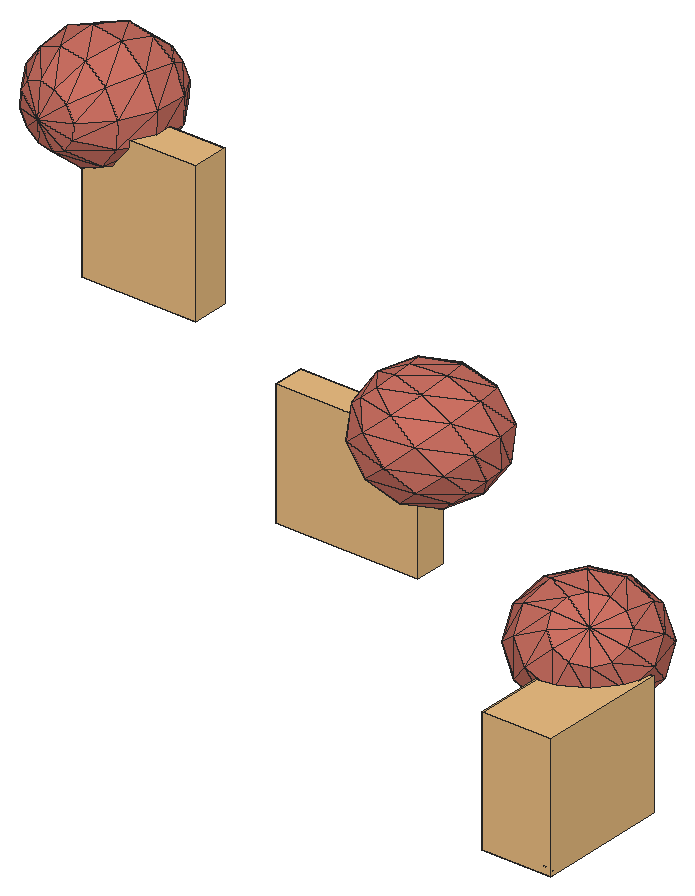
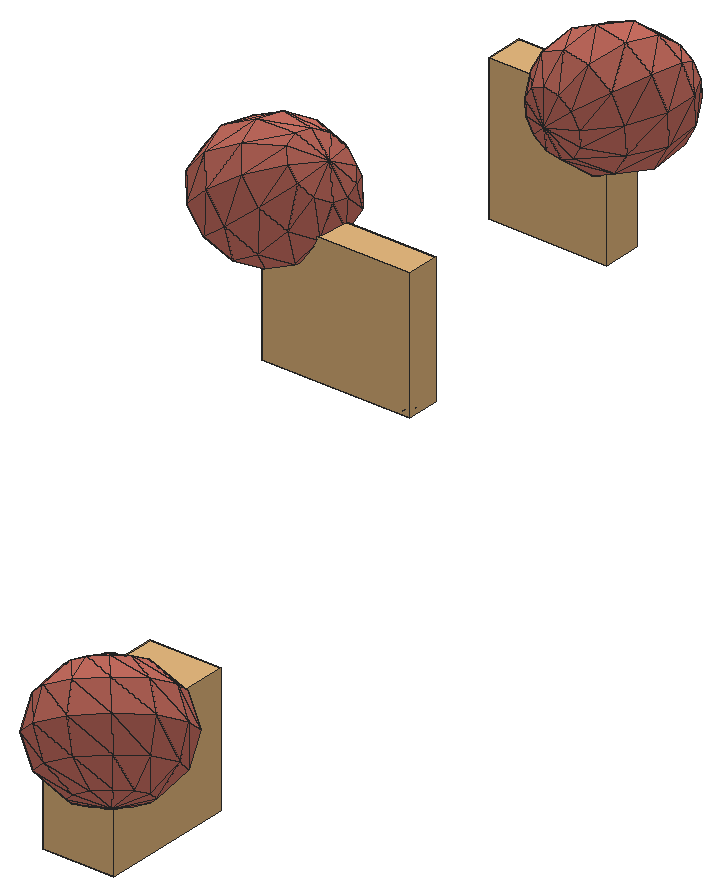
# SketchUp Ruby script. Lengths in inches.
U = 1.inch
M = Sketchup.active_model
def pt(a) = Geom::Point3d.new(a.map { |v| v * U })
def face(e, loops, mat)
  f = e.add_face(loops[0].map { |a| pt(a) })
  loops[1..].each { |l| e.add_face(l.map { |a| pt(a) }).erase! }
  f.material = f.back_material = mat if mat
  f
end
# faces: each face lists its corners as indices into pts; further lists are holes
def faces(e, pts, list, mat = nil) = list.each { |f| face(e, (f[0].is_a?(Array) ? f : [f]).map { |l| l.map { |i| pts[i] } }, mat) }
# xy, xz, yz: faces in a plane at the given z, y or x. An outline is a flat list of corners, or four numbers for a rectangle; further outlines are holes
def ring(l) = l.size == 4 ? [[l[0], l[1]], [l[2], l[1]], [l[2], l[3]], [l[0], l[3]]] : l.each_slice(2).to_a
def flat(e, list, mat, &to3) = list.each { |f| face(e, (f[0].is_a?(Array) ? f : [f]).map { |l| ring(l).map { |u, v| to3.(u, v) } }, mat) }
def xy(e, z, list, mat = nil) = flat(e, list, mat) { |x, y| [x, y, z] }
def xz(e, y, list, mat = nil) = flat(e, list, mat) { |x, z| [x, y, z] }
def yz(e, x, list, mat = nil) = flat(e, list, mat) { |y, z| [x, y, z] }
def lines(e, pts, list) = list.each { |a, b| e.add_line(pt(pts[a]), pt(pts[b])) }
# prism: a flat outline (further loops are holes) pulled along v
def prism(e, loops, v, mat = nil)
  f = face(e, loops, mat); d = Geom::Vector3d.new(v.map { |x| x * U })
  f.pushpull(f.normal.samedirection?(d) ? d.length : -d.length)
end
def box(e, o, s, mat = nil) = prism(e, [[o, [o[0] + s[0], o[1], o[2]], [o[0] + s[0], o[1] + s[1], o[2]], [o[0], o[1] + s[1], o[2]]]], [0, 0, s[2]], mat)
def at(x, y, z, deg = 0) = Geom::Transformation.translation(pt([x, y, z])) * Geom::Transformation.rotation(ORIGIN, Z_AXIS, deg.degrees)
def axes(o, x, y, z) = Geom::Transformation.new([*x, 0, *y, 0, *z, 0, *pt(o).to_a, 1])
def part(name) = M.definitions.add(name)
# library, detail: a bought-in or finely detailed component or shape, given as its bounding box
def library(name, o, s) = part(name).tap { |d| box(d.entities, o, s) }
def detail(e, o, s) = box(e.add_group.entities, o, s)
def put(e, d, t, mat = nil) = e.add_instance(d, t).tap { |i| i.material = mat if mat }
def group(e, t, mat = nil) = e.add_group.tap { |g| g.transformation = t; g.material = mat if mat }.entities
root = M.entities
M.materials.add("green").color = [174, 139, 102]
M.materials.add("vio").color = [206, 114, 100]
c1 = library("3DGeom~47_Defintion",[-132.29,-500,-408.57],[264.58,1000,817.14])
c2 = part("3DGeom~48_Defintion")
p = [[-103.8,487.39,-408.57],[-132.29,492.93,-365.46],[-123.73,496.1875,-348.87],[-103.8,487.39,-408.57],[-131.22,489.88,-384.15],[-132.29,492.93,-365.46],
  [-103.8,487.39,-408.57],[-120.79,487.85,-399.93],[-131.22,489.88,-384.15],[-103.8,487.39,-408.57],[-123.73,496.1875,-348.87],[-107.82,498.77,-338.8125],
  [-103.8,487.39,-408.57],[-107.82,498.77,-338.8125],[-88.83,500,-338],[-103.8,487.39,-408.57],[-60.34,494.46,-381.11],[-68.9,491.2,-397.7],
  [-103.8,487.39,-408.57],[-68.9,491.2,-397.7],[-84.8125,488.61,-407.76],[-103.8,487.39,-408.57],[-71.84,499.54,-346.64],[-61.42,497.51,-362.41],
  [-103.8,487.39,-408.57],[-61.42,497.51,-362.41],[-60.34,494.46,-381.11],[-103.8,487.39,-408.57],[-88.83,500,-338],[-71.84,499.54,-346.64],
  [91.01,-500,353.89],[109.71,-496.86,353.62],[124.82,-489.05,360.72],[62.5,-490.37,374.27],[91.01,-500,353.89],[67.8125,-469.79,401.48],
  [91.01,-500,353.89],[62.5,-490.37,374.27],[73.73,-497.625,361.44],[91.01,-500,353.89],[101.625,-458.84,408.31],[130.13,-468.47,387.93],
  [91.01,-500,353.89],[124.82,-489.05,360.72],[91.01,-500,353.89],[130.13,-468.47,387.93],[130.13,-468.47,387.93],[124.82,-489.05,360.72],
  [132.29,-478.66,373.28],[62.5,-490.37,374.27],[60.34,-480.18,388.92],[130.13,-468.47,387.93],[118.9,-461.21,400.75],[82.93,-461.98,408.57]]
faces(c2.entities,p,[[0,1,2],[3,4,5],[6,7,8],[9,10,11],[12,13,14],[15,16,17],[18,19,20],[21,22,23],
  [24,25,26],[27,28,29],[30,31,32],[33,34,35],[36,37,38],[35,39,40],[41,42,43],[40,44,45],
  [46,47,48],[49,35,50],[40,51,52],[35,40,53]],"green")
c3 = part("3DGeom~199_Defintion")
p = [[-69.55,-302.43,-360.84],[-338.74,-97.12,-366.25],[-102.46,-106.03,-485.67],[189.77,-256.61,-366.85],[161.26,-86.52,-474.95],[-343.46,97.57,-361.65],
  [-107.92,118.79,-480.36],[156.54,108.18,-470.35],[-323.15,264.7,-245.58],[-84.47,311.77,-346.33],[-323.15,264.7,-245.58],[-84.47,311.77,-346.33],
  [398.24,-142.03,-274.56],[398.24,-142.03,-274.56],[381.78,-43.83,-336.97],[381.78,-43.83,-336.97],[381.78,-43.83,-336.97],[379.05,68.57,-334.3125],
  [379.05,68.57,-334.3125],[176.85,275.3,-354.28],[-84.47,311.77,-346.33],[176.85,275.3,-354.28],[234.41,-356.52,-175.01],[-69.55,-302.43,-360.84],
  [189.77,-256.61,-366.85],[424.01,-199.72,-163.8],[234.41,-356.52,-175.01],[189.77,-256.61,-366.85],[189.77,-256.61,-366.85],[398.24,-142.03,-274.56],
  [-310.23,-267.21,-258.15],[-310.23,-267.21,-258.15],[-484.24,-62.19,-148.7],[-338.74,-97.12,-366.25],[-338.74,-97.12,-366.25],[-486.97,50.21,-146.04],
  [-338.74,-97.12,-366.25],[-343.46,97.57,-361.65],[-343.46,97.57,-361.65],[-475.25,146.71,-79.03],[-343.46,97.57,-361.65],[-323.15,264.7,-245.58],
  [-18,-417.8,-139.33],[-310.23,-267.21,-258.15],[-69.55,-302.43,-360.84],[234.41,-356.52,-175.01],[-69.55,-302.43,-360.84],[379.05,68.57,-334.3125],
  [176.85,275.3,-354.28],[390.78,165.07,-267.3],[390.78,165.07,-267.3],[176.85,275.3,-354.28],[216.77,370.09,-157.85],[176.85,275.3,-354.28],
  [-84.47,311.77,-346.33],[-38.375,421.22,-119.51],[176.85,275.3,-354.28],[216.77,370.09,-157.85],[-323.15,264.7,-245.58],[-283.23,359.48,-49.15],
  [381.78,-43.83,-336.97],[500,10.6,-108.7],[379.05,68.57,-334.3125],[413.82,219.79,-153.89],[-265.59,-367.12,-66.32],[-310.23,-267.21,-258.15],
  [-265.59,-367.12,-66.32],[-467.79,-160.39,-86.29],[-310.23,-267.21,-258.15],[-310.23,-267.21,-258.15],[-323.15,264.7,-245.58],[-452.2,201.43,34.38],
  [-323.15,264.7,-245.58],[-283.23,359.48,-49.15],[283.23,-359.48,49.15],[234.41,-356.52,-175.01],[452.2,-201.43,-34.38],[283.23,-359.48,49.15],
  [265.59,367.12,66.32],[216.77,370.09,-157.85],[18,417.8,139.33],[265.59,367.12,66.32],[216.77,370.09,-157.85],[442.01,218.08,-24.47],
  [-500,-10.6,108.7],[38.375,-421.22,119.51],[283.23,-359.48,49.15],[-234.41,356.52,175.02],[475.25,-146.71,79.03],[486.97,-50.21,146.04],
  [484.24,62.19,148.7],[467.79,160.39,86.29],[-265.59,-367.12,-66.32],[-442.01,-218.08,24.47],[-216.77,-370.09,157.85],[-216.77,-370.09,157.85],
  [-265.59,-367.12,-66.32],[-283.23,359.48,-49.15],[-424.01,199.72,163.8],[-283.23,359.48,-49.15],[-234.41,356.52,175.02],[310.23,267.21,258.15],
  [-216.77,-370.09,157.85],[-413.82,-219.79,153.89],[323.15,-264.7,245.59],[283.23,-359.48,49.15],[323.15,-264.7,245.59],[265.59,367.12,66.32],
  [69.55,302.43,360.84],[310.23,267.21,258.15],[265.59,367.12,66.32],[69.55,302.43,360.84],[338.74,97.12,366.25],[-390.78,-165.07,267.3],
  [-390.78,-165.07,267.3],[-379.05,-68.57,334.3125],[-379.05,-68.57,334.3125],[-381.78,43.83,336.97],[-381.78,43.83,336.97],[-398.24,142.03,274.56],
  [-398.24,142.03,274.56],[84.47,-311.77,346.34],[323.15,-264.7,245.59],[84.47,-311.77,346.34],[-189.77,256.61,366.85],[-189.77,256.61,366.85],
  [69.55,302.43,360.84],[343.46,-97.57,361.65],[-176.85,-275.3,354.28],[-216.77,-370.09,157.85],[-176.85,-275.3,354.28],[-390.78,-165.07,267.3],
  [84.47,-311.77,346.34],[-176.85,-275.3,354.28],[-234.41,356.52,175.02],[-398.24,142.03,274.56],[-234.41,356.52,175.02],[-398.24,142.03,274.56],
  [-189.77,256.61,366.85],[343.46,-97.57,361.65],[84.47,-311.77,346.34],[323.15,-264.7,245.59],[310.23,267.21,258.15],[102.46,106.03,485.67],
  [338.74,97.12,366.25],[310.23,267.21,258.15],[69.55,302.43,360.84],[-156.54,-108.17,470.35],[-390.78,-165.07,267.3],[-176.85,-275.3,354.28],
  [-379.05,-68.57,334.3125],[-189.77,256.61,366.85],[-398.24,142.03,274.56],[-381.78,43.83,336.97],[-161.26,86.52,474.95],[107.92,-118.79,480.36],
  [343.46,-97.57,361.65],[338.74,97.12,366.25],[343.46,-97.57,361.65],[338.74,97.12,366.25]]
faces(c3.entities,p,[[0,1,2],[3,0,2],[3,2,4],[2,1,5],[2,5,6],[4,2,6],[4,6,7],[6,5,8],
  [7,6,9],[6,10,11],[12,3,4],[13,4,14],[15,4,7],[16,7,17],[18,7,19],[7,20,21],
  [22,23,24],[25,26,27],[25,28,29],[0,30,1],[31,32,33],[34,32,35],[36,35,37],[38,35,39],
  [40,39,41],[42,43,44],[45,42,46],[47,48,49],[50,51,52],[53,54,55],[56,55,57],[54,58,59],
  [54,59,55],[29,60,61],[60,62,61],[62,50,61],[25,29,61],[50,63,61],[50,52,63],[42,64,65],
  [66,67,68],[69,67,32],[70,39,71],[72,71,73],[74,42,75],[76,77,26],[76,26,25],[76,25,61],
  [63,52,78],[79,80,81],[82,55,80],[63,83,61],[63,78,83],[32,67,84],[35,32,84],[39,35,84],
  [85,64,42],[86,85,42],[55,59,87],[55,87,80],[88,76,61],[89,88,61],[90,89,61],[83,91,61],
  [91,90,61],[92,93,67],[67,93,84],[71,39,84],[85,94,64],[95,93,96],[97,71,98],[99,98,100],
  [88,77,76],[83,101,91],[83,78,101],[102,103,93],[93,103,84],[98,71,84],[104,85,105],[88,106,77],
  [107,108,109],[110,80,111],[89,106,88],[91,112,90],[91,101,112],[103,113,84],[114,115,84],[116,117,84],
  [118,119,84],[120,98,84],[121,94,85],[122,123,85],[80,87,124],[80,125,126],[89,127,106],[90,127,89],
  [90,112,127],[128,103,129],[130,131,103],[132,133,94],[134,98,135],[136,137,138],[139,140,141],[142,143,144],
  [145,146,143],[147,148,149],[147,150,148],[151,152,153],[154,150,147],[154,153,150],[151,153,154],[155,149,140],
  [156,155,140],[155,147,149],[146,151,154],[146,154,143],[157,155,158],[159,143,155],[143,147,155],[143,154,147]],"vio")
c4 = part("3DGeom~205_Defintion")
p = [[47.4,99.55,-486.18],[46.74,-121.12,-479.41],[-173.66,-85.23,-460.58],[170.15,120.28,-450.94],[-79.85,120.28,-475.32],[35.36,293.55,-362.6875],
  [33.56,-309.34,-344.18],[-220.94,-267.89,-322.44],[259.35,-85.23,-418.37],[-342.79,12.83,-366.9375],[-177.49,176.89,-421.25],[-416.23,-154.67,-214.3],
  [-416.23,-154.67,-214.3],[255.52,176.89,-379.03],[-415.33,146.77,-223.56],[-415.33,146.77,-223.56],[-219.38,254.22,-338.47],[279.06,-267.9,-273.69],
  [407.21,12.83,-293.82],[279.06,-267.9,-273.69],[259.35,-85.23,-418.37],[407.21,12.83,-293.82],[280.62,254.22,-289.72],[407.21,12.83,-293.82],
  [255.52,176.89,-379.03],[280.62,254.22,-289.72],[-342.79,12.83,-366.9375],[-416.23,-154.67,-214.3],[-500,0,-48.75],[-342.79,12.83,-366.9375],
  [-415.33,146.77,-223.56],[-194.27,331.56,-249.16],[238.74,331.56,-206.94],[-194.27,331.56,-249.16],[-108.91,388.17,-177.25],[35.36,293.55,-362.6875],
  [13.85,408.89,-142.01],[35.36,293.55,-362.6875],[141.09,388.17,-152.875],[35.36,293.55,-362.6875],[238.74,331.56,-206.94],[35.36,293.55,-362.6875],
  [33.56,-309.34,-344.18],[11.38,-414.67,-116.72],[-209.02,-378.78,-97.9],[279.06,-267.9,-273.69],[33.56,-309.34,-344.18],[33.56,-309.34,-344.18],
  [-209.02,-378.78,-97.9],[-220.94,-267.89,-322.44],[-219.38,254.22,-338.47],[-371.85,280.72,-68.87],[-219.38,254.22,-338.47],[-371.85,280.72,-68.87],
  [-194.27,331.56,-249.16],[-220.94,-267.89,-322.44],[-209.02,-378.78,-97.9],[-378.15,-280.72,-4.25],[-220.94,-267.89,-322.44],[407.21,12.83,-293.82],
  [449.79,-154.67,-129.87],[279.06,-267.9,-273.69],[450.69,146.77,-139.125],[407.21,12.83,-293.82],[280.62,254.22,-289.72],[407.21,12.83,-293.82],
  [238.74,331.56,-206.94],[280.62,254.22,-289.72],[279.06,-267.9,-273.69],[223.99,-378.78,-55.68],[223.99,-378.78,-55.68],[279.06,-267.9,-273.69],
  [-371.85,280.72,-68.87],[-223.99,378.78,55.68],[-449.79,154.67,129.87],[-371.85,280.72,-68.87],[-450.69,-146.77,139.13],[238.74,331.56,-206.94],
  [378.15,280.72,4.25],[378.15,280.72,4.25],[238.74,331.56,-206.94],[-11.38,414.67,116.72],[209.02,378.78,97.9],[378.15,280.72,4.25],
  [500,0,48.75],[371.85,-280.72,68.87],[223.99,-378.78,-55.68],[-141.09,-388.17,152.875],[-209.02,-378.78,-97.9],[-13.85,-408.89,142.01],
  [-209.02,-378.78,-97.9],[-238.74,-331.56,206.94],[-209.02,-378.78,-97.9],[-238.74,-331.56,206.94],[-378.15,-280.72,-4.25],[-371.85,280.72,-68.87],
  [-279.06,267.9,273.69],[-371.85,280.72,-68.87],[-279.06,267.9,273.69],[-223.99,378.78,55.68],[108.91,-388.17,177.25],[371.85,-280.72,68.87],
  [-407.21,-12.83,293.82],[-238.74,-331.56,206.94],[-280.62,-254.22,289.72],[416.23,154.67,214.31],[209.02,378.78,97.9],[415.33,-146.77,223.56],
  [-279.06,267.9,273.69],[-33.56,309.34,344.18],[371.85,-280.72,68.87],[194.27,-331.56,249.16],[194.27,-331.56,249.16],[209.02,378.78,97.9],
  [220.94,267.89,322.44],[220.94,267.89,322.44],[220.94,267.89,322.44],[-259.35,85.23,418.37],[-259.35,85.23,418.37],[-279.06,267.9,273.69],
  [-255.52,-176.89,379.03],[-255.52,-176.89,379.03],[-35.36,-293.55,362.6875],[-238.74,-331.56,206.94],[-280.62,-254.22,289.72],[-238.74,-331.56,206.94],
  [-35.36,-293.55,362.6875],[342.79,-12.83,366.9375],[220.94,267.89,322.44],[342.79,-12.83,366.9375],[416.23,154.67,214.31],[219.38,-254.22,338.47],
  [194.27,-331.56,249.16],[342.79,-12.83,366.9375],[219.38,-254.22,338.47],[415.33,-146.77,223.56],[194.27,-331.56,249.16],[219.38,-254.22,338.47],
  [-35.36,-293.55,362.6875],[-279.06,267.9,273.69],[-259.35,85.23,418.37],[-46.74,121.12,479.41],[-279.06,267.9,273.69],[-33.56,309.34,344.18],
  [-255.52,-176.89,379.03],[-280.62,-254.22,289.72],[-35.36,-293.55,362.6875],[-407.21,-12.83,293.82],[-170.15,-120.28,450.94],[-407.21,-12.83,293.82],
  [220.94,267.89,322.44],[173.66,85.23,460.58],[342.79,-12.83,366.9375],[-33.56,309.34,344.18],[220.94,267.89,322.44],[219.38,-254.22,338.47],
  [177.49,-176.89,421.25],[-35.36,-293.55,362.6875],[342.79,-12.83,366.9375],[219.38,-254.22,338.47],[-33.56,309.34,344.18],[-35.36,-293.55,362.6875],
  [-47.4,-99.55,486.18],[-35.36,-293.55,362.6875],[79.85,-120.28,475.32],[-35.36,-293.55,362.6875],[-35.36,-293.55,362.6875],[342.79,-12.83,366.9375]]
faces(c4.entities,p,[[0,1,2],[3,1,0],[0,2,4],[0,4,5],[3,0,5],[1,6,7],[8,6,1],[1,7,2],
  [3,8,1],[4,2,9],[4,9,10],[4,10,5],[2,7,11],[2,12,9],[13,8,3],[13,3,5],
  [10,9,14],[10,15,16],[10,16,5],[8,17,6],[18,19,20],[13,21,8],[22,23,24],[25,13,5],
  [26,27,28],[29,28,30],[16,31,5],[32,25,5],[33,34,35],[34,36,37],[36,38,39],[38,40,41],
  [42,43,44],[45,43,46],[47,48,49],[50,30,51],[52,53,54],[55,56,57],[58,57,27],[59,60,61],
  [62,60,63],[64,62,65],[66,62,67],[68,69,43],[60,70,71],[33,72,73],[33,73,34],[30,28,74],
  [30,74,75],[27,57,76],[27,76,28],[77,78,62],[38,79,80],[34,73,81],[34,81,36],[38,82,83],
  [36,82,38],[36,81,82],[62,84,60],[78,84,62],[60,85,86],[84,85,60],[43,87,88],[43,89,87],
  [69,89,43],[90,87,91],[92,93,94],[95,74,96],[97,98,99],[69,100,89],[101,100,69],[28,76,102],
  [28,102,74],[57,103,104],[57,104,76],[78,105,84],[106,105,78],[84,107,85],[105,107,84],[73,108,109],
  [73,109,81],[110,111,100],[107,112,85],[113,114,105],[81,115,82],[81,109,116],[74,102,117],[74,118,119],
  [76,104,120],[76,121,102],[87,89,122],[89,100,122],[123,87,122],[100,111,122],[124,125,126],[105,127,107],
  [128,129,130],[107,131,132],[133,134,135],[136,137,138],[139,140,141],[142,141,143],[144,145,146],[147,144,148],
  [149,148,140],[150,151,152],[153,151,154],[155,156,157],[158,156,159],[160,141,151],[148,144,161],[162,148,163],
  [164,162,165],[156,164,166],[151,156,167],[140,148,162],[140,162,141],[151,164,156],[141,164,151],[141,162,164]],"vio")
c5 = library("3DGeom~59_Defintion",[-108.27,-437.54,-500],[216.54,875.08,1000])
c6 = part("3DGeom~60_Defintion")
p = [[-48.9,-398.48,-495.36],[-85.15,-397.34,-497.61],[-66.68,-395.0625,-500],[-105.49,-415.16,-476],[-99.36,-404.6875,-488.82],[-85.15,-397.34,-497.61],
  [-105.49,-415.16,-476],[-85.15,-397.34,-497.61],[-32.98,-417.45,-471.51],[-105.49,-415.16,-476],[-32.98,-417.45,-471.51],[-36.5625,-406.68,-484.93],
  [-53.33,-435.27,-449.91],[-105.49,-415.16,-476],[-32.98,-417.45,-471.51],[-89.58,-434.125,-452.15],[-105.49,-415.16,-476],[-53.33,-435.27,-449.91],
  [-105.49,-415.16,-476],[-89.58,-434.125,-452.15],[-101.92,-425.93,-462.58],[-53.33,-435.27,-449.91],[-32.98,-417.45,-471.51],[-39.12,-427.92,-458.69],
  [-89.58,-434.125,-452.15],[-53.33,-435.27,-449.91],[-71.8,-437.54,-447.51],[44.63,425.16,482.47],[105.29,413.34,449.94],[94.58,425.52,444.15],
  [44.63,425.16,482.47],[94.58,425.52,444.15],[79.01,434.375,445.83],[44.63,425.16,482.47],[79.01,434.375,445.83],[62.76,437.54,454.55],
  [44.63,425.16,482.47],[108.27,401.11,461.67],[105.29,413.34,449.94],[44.63,425.16,482.47],[62.76,437.54,454.55],[50.17,434.17,467.96],
  [44.63,425.16,482.47],[102.73,392.1,476.1875],[108.27,401.11,461.67],[44.63,425.16,482.47],[90.15,388.73,489.6],[102.73,392.1,476.1875],
  [44.63,425.16,482.47],[73.89,391.89,498.32],[90.15,388.73,489.6],[44.63,425.16,482.47],[58.33,400.75,500],[73.89,391.89,498.32],
  [44.63,425.16,482.47],[47.61,412.93,494.2]]
faces(c6.entities,p,[[0,1,2],[3,4,5],[0,6,7],[8,9,0],[10,0,11],[12,13,14],[15,16,17],[18,19,20],
  [21,22,23],[24,25,26],[27,28,29],[30,31,32],[33,34,35],[36,37,38],[39,40,41],[42,43,44],
  [45,46,47],[48,49,50],[51,52,53],[54,55,52]],"green")
c7 = library("3DGeom~57_Defintion",[-500,-478.45,-265.375],[1000,956.89,530.75])
c8 = part("3DGeom~58_Defintion")
p = [[-465.47,464.9,-258.6875],[-477.89,451.53,-263.24],[-489.74,438.22,-257.15],[-465.47,464.9,-258.6875],[-497.83,428.53,-242.0625],[-500,425.07,-222.01],
  [-465.47,464.9,-258.6875],[-500,425.07,-222.01],[-495.67,428.76,-202.375],[-465.47,464.9,-258.6875],[-489.74,438.22,-257.15],[-497.83,428.53,-242.0625],
  [-465.47,464.9,-258.6875],[-495.67,428.76,-202.375],[-485.99,438.61,-188.41],[-465.47,464.9,-258.6875],[-485.99,438.61,-188.41],[-473.5625,451.98,-183.86],
  [-465.47,464.9,-258.6875],[-473.5625,451.98,-183.86],[-461.72,465.3,-189.95],[-465.47,464.9,-258.6875],[-453.625,474.98,-205.04],[-451.46,478.44,-225.09],
  [-465.47,464.9,-258.6875],[-451.46,478.44,-225.09],[-455.79,474.75,-244.72],[-465.47,464.9,-258.6875],[-461.72,465.3,-189.95],[-453.625,474.98,-205.04],
  [492.22,-453.97,197.65],[460.87,-474.71,197.28],[477.9,-465.75,192.59],[460.87,-474.71,197.28],[436.46,-475.96,228.62],[445.7,-478.45,210.47],
  [460.87,-474.71,197.28],[492.22,-453.97,197.65],[436.46,-475.96,228.62],[436.46,-475.96,228.62],[492.22,-453.97,197.65],[443.4,-456.48,260.3125],
  [443.4,-456.48,260.3125],[492.22,-453.97,197.65],[474.74,-435.74,260.68],[474.74,-435.74,260.68],[492.22,-453.97,197.65],[499.15,-434.48,229.35],
  [492.22,-453.97,197.65],[500,-442.52,211.1],[499.15,-434.48,229.35],[436.46,-475.96,228.62],[443.4,-456.48,260.3125],[435.61,-467.92,246.86],
  [474.74,-435.74,260.68],[499.15,-434.48,229.35],[489.91,-432,247.49],[443.4,-456.48,260.3125],[474.74,-435.74,260.68],[457.72,-444.7,265.375]]
faces(c8.entities,p,[[0,1,2],[3,4,5],[6,7,8],[9,10,11],[12,13,14],[15,16,17],[18,19,20],[21,22,23],
  [24,25,26],[27,28,29],[30,31,32],[33,34,35],[36,37,38],[39,40,41],[42,43,44],[45,46,47],
  [48,49,50],[51,52,53],[54,55,56],[57,58,59]],"green")
c9 = part("3DGeom~204_Defintion")
p = [[-12.5,-12.78,-500],[-167.87,-176.1875,-423.23],[-275,-119.8,-393.5],[139.12,-146.19,-448.74],[321.29,0,-383.61],[-198.05,84.89,-448.51],
  [146.22,154.06,-442.79],[216.18,-279.61,-308.47],[-80.33,-253.22,-393.64],[410.28,-154.06,-221.63],[410.28,-154.06,-221.63],[-373.01,-99.16,-312.41],
  [-373.01,-99.16,-312.41],[-367.81,120.64,-308.0625],[-68.03,266.84,-383.34],[-367.81,120.64,-308.0625],[-68.03,266.84,-383.34],[417.375,146.19,-215.68],
  [417.375,146.19,-215.68],[265.76,279.61,-266.94],[265.76,279.61,-266.94],[-68.03,266.84,-383.34],[-278.26,-292.39,-233.06],[-278.26,-292.39,-233.06],
  [-35.84,-330.25,-312.65],[-278.26,-292.39,-233.06],[-373.01,-99.16,-312.41],[-275,-119.8,-393.5],[-278.26,-292.39,-233.06],[494.4375,12.78,-75.41],
  [410.28,-154.06,-221.63],[321.29,0,-383.61],[321.29,0,-383.61],[417.375,146.19,-215.68],[-68.03,266.84,-383.34],[-367.81,120.64,-308.0625],
  [-264.06,308.11,-221.16],[80.21,377.28,-215.45],[-68.03,266.84,-383.34],[-264.06,308.11,-221.16],[265.76,279.61,-266.94],[-68.03,266.84,-383.34],
  [80.21,377.28,-215.45],[-35.84,-330.25,-312.65],[-46.32,-386.64,-201.97],[-278.26,-292.39,-233.06],[198.04,-377.28,-116.76],[-35.84,-330.25,-312.65],
  [198.04,-377.28,-116.76],[-35.84,-330.25,-312.65],[216.18,-279.61,-308.47],[-435.64,-119.8,-201.7],[-278.26,-292.39,-233.06],[-367.81,120.64,-308.0625],
  [389.33,-266.84,-0.27],[198.04,-377.28,-116.76],[216.18,-279.61,-308.47],[216.18,-279.61,-308.47],[-476.3,84.89,-116.29],[-264.06,308.11,-221.16],
  [401.625,253.22,10.03],[265.76,279.61,-266.94],[265.76,279.61,-266.94],[314.09,330.25,-19.5625],[314.09,330.25,-19.5625],[265.76,279.61,-266.94],
  [-108.95,-407.27,-91.25],[-206.96,-386.64,-10.17],[-314.09,-330.25,19.5625],[-314.09,-330.25,19.5625],[-401.625,-253.22,-10.03],[-278.26,-292.39,-233.06],
  [-446.12,-176.1875,-91.02],[-278.26,-292.39,-233.06],[-278.26,-292.39,-233.06],[476.3,-84.89,116.29],[-264.06,308.11,-221.16],[-389.33,266.84,0.27],
  [-89.55,413.03,-75],[-389.33,266.84,0.27],[446.12,176.1875,91.02],[206.96,386.64,10.17],[89.55,-413.03,75],[198.04,-377.28,-116.76],
  [264.06,-308.11,221.16],[198.04,-377.28,-116.76],[264.06,-308.11,221.16],[198.04,-377.28,-116.76],[389.33,-266.84,-0.27],[-494.4375,-12.78,75.41],
  [-80.21,-377.28,215.45],[435.64,119.8,201.7],[-389.33,266.84,0.27],[-198.04,377.28,116.76],[108.95,407.27,91.25],[314.09,330.25,-19.5625],
  [278.26,292.39,233.06],[278.26,292.39,233.06],[-265.76,-279.61,266.94],[-265.76,-279.61,266.94],[-417.375,-146.19,215.68],[-314.09,-330.25,19.5625],
  [-417.375,-146.19,215.68],[367.81,-120.64,308.0625],[264.06,-308.11,221.16],[367.81,-120.64,308.0625],[-410.28,154.06,221.63],[-198.04,377.28,116.76],
  [-410.28,154.06,221.63],[278.26,292.39,233.06],[-417.375,-146.19,215.68],[-314.09,-330.25,19.5625],[-265.76,-279.61,266.94],[68.03,-266.84,383.34],
  [68.03,-266.84,383.34],[264.06,-308.11,221.16],[-410.28,154.06,221.63],[-417.375,-146.19,215.68],[46.32,386.64,201.97],[278.26,292.39,233.06],
  [373.01,99.16,312.41],[367.81,-120.64,308.0625],[-198.04,377.28,116.76],[-410.28,154.06,221.63],[-216.18,279.61,308.47],[-216.18,279.61,308.47],
  [-216.18,279.61,308.47],[35.84,330.25,312.65],[35.84,330.25,312.65],[278.26,292.39,233.06],[-146.22,-154.06,442.79],[-265.76,-279.61,266.94],
  [-80.21,-377.28,215.45],[-80.21,-377.28,215.45],[68.03,-266.84,383.34],[-321.29,0,383.61],[-417.375,-146.19,215.68],[-410.28,154.06,221.63],
  [-417.375,-146.19,215.68],[-321.29,0,383.61],[198.05,-84.89,448.51],[264.06,-308.11,221.16],[367.81,-120.64,308.0625],[-216.18,279.61,308.47],
  [-410.28,154.06,221.63],[275,119.8,393.5],[167.87,176.1875,423.23],[275,119.8,393.5],[278.26,292.39,233.06],[80.33,253.22,393.64],
  [278.26,292.39,233.06],[35.84,330.25,312.65],[278.26,292.39,233.06],[275,119.8,393.5],[275,119.8,393.5],[373.01,99.16,312.41],
  [-139.12,146.19,448.74],[12.5,12.78,500],[275,119.8,393.5]]
faces(c9.entities,p,[[0,1,2],[3,1,0],[4,3,0],[0,2,5],[6,0,5],[4,0,6],[7,8,3],[9,7,3],
  [3,8,1],[10,3,4],[5,2,11],[5,12,13],[14,5,15],[6,5,16],[17,4,6],[18,6,19],
  [20,6,21],[2,1,22],[1,8,23],[8,24,25],[7,24,8],[26,27,28],[29,30,31],[29,32,33],
  [34,35,36],[37,38,39],[40,41,42],[43,44,45],[46,44,47],[48,49,50],[51,26,52],[53,26,51],
  [54,55,56],[54,57,30],[53,51,58],[59,53,58],[60,33,61],[60,62,63],[64,65,37],[66,67,45],
  [44,66,45],[67,68,45],[69,70,71],[70,72,73],[72,51,74],[75,54,30],[75,30,29],[76,58,77],
  [78,39,79],[37,39,78],[80,29,33],[80,33,60],[64,37,81],[81,37,78],[82,66,44],[82,44,83],
  [58,51,72],[84,82,85],[86,87,88],[58,72,89],[77,58,89],[90,66,82],[90,67,66],[89,72,70],
  [91,75,29],[91,29,80],[78,92,93],[94,78,93],[81,78,94],[60,95,96],[64,81,97],[98,68,67],
  [99,67,90],[100,70,101],[89,70,102],[103,104,54],[105,54,75],[77,89,106],[107,77,108],[80,60,96],
  [81,94,109],[110,111,112],[113,90,82],[114,82,115],[116,89,117],[91,80,96],[94,118,119],[94,93,118],
  [120,121,75],[120,75,91],[122,123,124],[118,93,125],[120,91,96],[118,126,127],[118,128,129],[130,131,132],
  [130,133,134],[135,136,131],[137,138,139],[140,134,141],[140,141,142],[143,144,135],[145,120,96],[146,147,148],
  [149,146,150],[151,149,152],[135,131,130],[153,140,142],[154,142,155],[143,135,156],[151,143,156],[151,156,149],
  [157,130,134],[157,134,140],[156,135,130],[146,140,158],[149,156,157],[149,157,146],[146,157,140],[156,130,157]],"vio")
g1 = group(root,at(15.3125,38.42,26.21))
put(g1,c1,axes([-1.33,0.32,11.7],[0,0.0004,0],[0,0,-0.0004],[-0.0004,0,0]),"green")
put(g1,c2,axes([-1.33,0.32,11.7],[0,0.0004,0],[0,0,-0.0004],[-0.0004,0,0]),"green")
g2 = group(root,at(15.3125,38.42,26.21))
put(g2,c3,axes([-1.51,0.37,11.92],[0,0.00038,0],[0,0,-0.00038],[-0.00038,0,0]),"vio")
g3 = group(root,at(15.3125,38.42,26.21))
put(g3,c4,axes([-0.58,0.38,11.37],[0,0.00039,0],[0,0,-0.00039],[-0.00039,0,0]),"vio")
g4 = group(root,at(15.3125,38.42,26.21))
put(g4,c5,axes([-0.81,0.41,11.17],[0,0.00041,0],[0,0,-0.00041],[-0.00041,0,0]),"green")
put(g4,c6,axes([-0.81,0.41,11.17],[0,0.00041,0],[0,0,-0.00041],[-0.00041,0,0]),"green")
g5 = group(root,at(15.3125,38.42,26.21))
put(g5,c7,axes([-0.65,0.96,10.24],[0,0.00037,0],[0,0,-0.00037],[-0.00037,0,0]),"green")
put(g5,c8,axes([-0.65,0.96,10.24],[0,0.00037,0],[0,0,-0.00037],[-0.00037,0,0]),"green")
g6 = group(root,at(15.3125,38.42,26.21))
put(g6,c9,axes([-0.75,1.16,10.43],[0,0.00039,0],[0,0,-0.00039],[-0.00039,0,0]),"vio")
